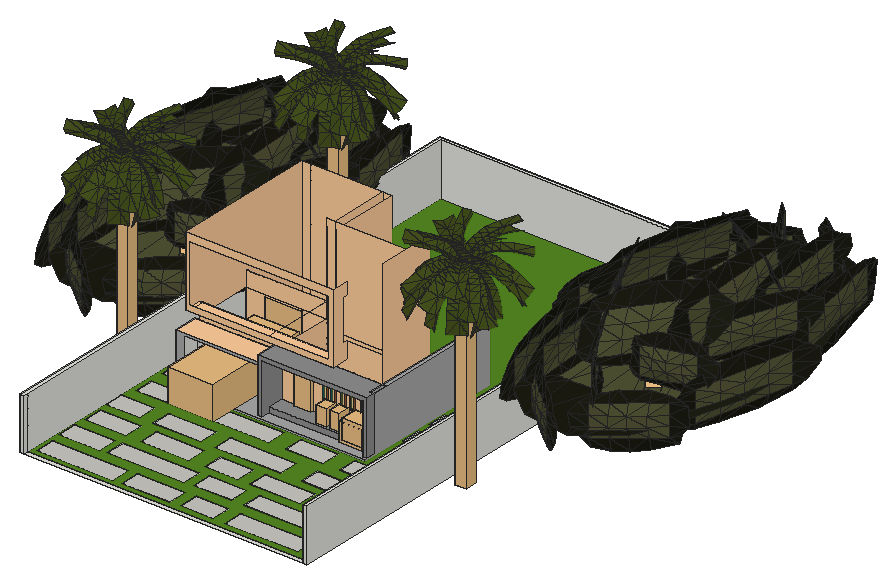
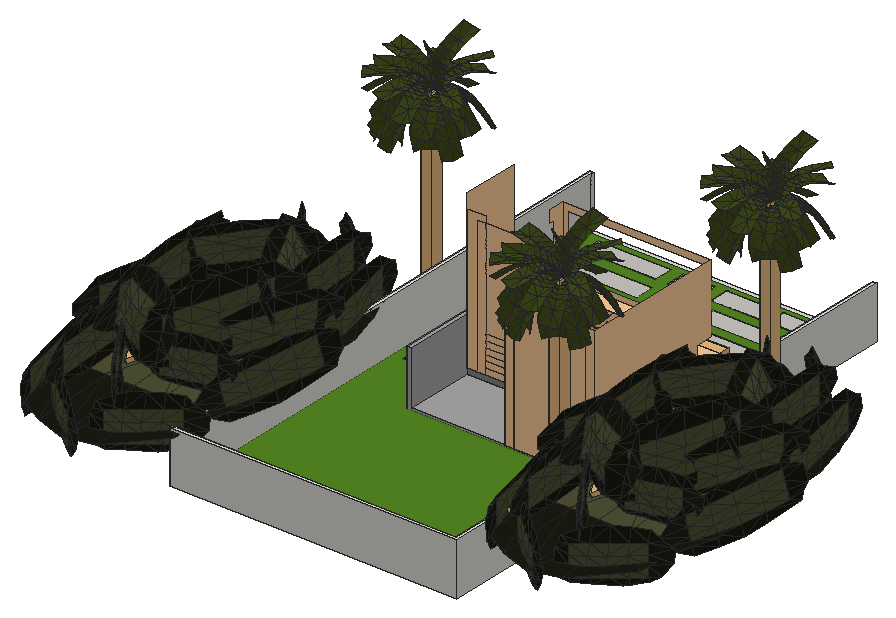
# SketchUp Ruby script. Lengths in inches.
U = 1.inch
M = Sketchup.active_model
def pt(a) = Geom::Point3d.new(a.map { |v| v * U })
def face(e, loops, mat)
  f = e.add_face(loops[0].map { |a| pt(a) })
  loops[1..].each { |l| e.add_face(l.map { |a| pt(a) }).erase! }
  f.material = f.back_material = mat if mat
  f
end
# faces: each face lists its corners as indices into pts; further lists are holes
def faces(e, pts, list, mat = nil) = list.each { |f| face(e, (f[0].is_a?(Array) ? f : [f]).map { |l| l.map { |i| pts[i] } }, mat) }
# xy, xz, yz: faces in a plane at the given z, y or x. An outline is a flat list of corners, or four numbers for a rectangle; further outlines are holes
def ring(l) = l.size == 4 ? [[l[0], l[1]], [l[2], l[1]], [l[2], l[3]], [l[0], l[3]]] : l.each_slice(2).to_a
def flat(e, list, mat, &to3) = list.each { |f| face(e, (f[0].is_a?(Array) ? f : [f]).map { |l| ring(l).map { |u, v| to3.(u, v) } }, mat) }
def xy(e, z, list, mat = nil) = flat(e, list, mat) { |x, y| [x, y, z] }
def xz(e, y, list, mat = nil) = flat(e, list, mat) { |x, z| [x, y, z] }
def yz(e, x, list, mat = nil) = flat(e, list, mat) { |y, z| [x, y, z] }
def lines(e, pts, list) = list.each { |a, b| e.add_line(pt(pts[a]), pt(pts[b])) }
# prism: a flat outline (further loops are holes) pulled along v
def prism(e, loops, v, mat = nil)
  f = face(e, loops, mat); d = Geom::Vector3d.new(v.map { |x| x * U })
  f.pushpull(f.normal.samedirection?(d) ? d.length : -d.length)
end
def box(e, o, s, mat = nil) = prism(e, [[o, [o[0] + s[0], o[1], o[2]], [o[0] + s[0], o[1] + s[1], o[2]], [o[0], o[1] + s[1], o[2]]]], [0, 0, s[2]], mat)
def at(x, y, z, deg = 0) = Geom::Transformation.translation(pt([x, y, z])) * Geom::Transformation.rotation(ORIGIN, Z_AXIS, deg.degrees)
def axes(o, x, y, z) = Geom::Transformation.new([*x, 0, *y, 0, *z, 0, *pt(o).to_a, 1])
def part(name) = M.definitions.add(name)
# library, detail: a bought-in or finely detailed component or shape, given as its bounding box
def library(name, o, s) = part(name).tap { |d| box(d.entities, o, s) }
def detail(e, o, s) = box(e.add_group.entities, o, s)
def put(e, d, t, mat = nil) = e.add_instance(d, t).tap { |i| i.material = mat if mat }
def group(e, t, mat = nil) = e.add_group.tap { |g| g.transformation = t; g.material = mat if mat }.entities
root = M.entities
M.materials.add("Brick_14_1K").color = [201, 199, 193]
M.materials.add("C02_Golden_Beige").color = [255, 205, 155]
M.materials.add("Glass_Basic_01").color = [176, 211, 103]
M.materials["Glass_Basic_01"].alpha = 0.25
M.materials.add("M03_Pewter_Shine").color = [168, 168, 168]
M.materials.add("M04_Stone_Frost").color = [142, 142, 142]
M.materials.add("Oak100_bottom").color = [27, 27, 17]
M.materials.add("Oak100_middle2").color = [80, 82, 52]
M.materials.add("Oak100_rs").color = [30, 31, 20]
M.materials.add("Oak100_top").color = [27, 27, 19]
M.materials.add("[0042_Sienna]").color = [160, 82, 45]
M.materials.add("[Color_004]").color = [176, 174, 161]
M.materials.add("[Color_F17]").color = [77, 130, 25]
M.materials["[Color_F17]"].alpha = 0.96
M.materials.add("[Color_H12]").color = [30, 153, 153]
M.materials.add("[Color_H17]").color = [20, 102, 102]
M.materials.add("[Color_H21]").color = [0, 51, 51]
M.materials.add("oak100_ls").color = [26, 27, 18]
M.materials.add("palmleaf").color = [66, 78, 27]
c1 = part("oak301branch")
detail(c1.entities,[0,-0.89,-1.57],[71.59,23.14,154.31])
c2 = part("center")
p = [[110.38,-8.75,48.08],[55.19,-7.5,48.08],[55.19,0,0.51],[110.38,0,0.51],[165.57,0,0.51],[165.57,-5.5,48.08],
  [0,0,48.08],[0,0,0.51],[220.76,0,0.51],[220.76,0,48.08],[110.38,-9,96.42],[55.19,-8,96.42],
  [165.57,-5,96.42],[0,0,96.42],[220.76,0,96.42],[110.38,0,144.75],[55.19,0,144.75],[165.57,0,144.75],
  [0,0,144.75],[220.76,0,144.75]]
faces(c2.entities,p,[[0,1,2],[0,2,3],[0,3,4],[0,4,5],[1,6,7],[1,7,2],[5,4,8],[5,8,9],
  [0,10,11],[0,12,10],[0,11,1],[0,5,12],[1,11,13],[1,13,6],[12,5,9],[12,9,14],
  [10,15,16],[10,16,11],[10,12,17],[10,17,15],[11,16,18],[11,18,13],[12,14,19],[12,19,17]],"Oak100_middle2")
c3 = part("leftside")
p = [[-0.5,8.25,24.35],[16,4.5,0],[47.5,0,0],[47.5,0,48.08],[-0.01,12.25,116.11],[47.5,0,96.42],
  [47.5,0,143.74],[16,6.25,143.74]]
faces(c3.entities,p,[[0,1,2],[0,2,3],[4,0,3],[4,3,5],[4,5,6],[4,6,7]],"oak100_ls")
c4 = part("rightside")
p = [[31.5,6,0],[63.6875,8.75,48.09],[0,0,48.08],[0,0,0],[62.93,15,107.53],[0,0,96.42],
  [0,0,144.75],[31.5,9.125,144.75]]
faces(c4.entities,p,[[0,1,2],[0,2,3],[1,4,5],[1,5,2],[4,6,5],[4,7,6]],"Oak100_rs")
c5 = part("top")
p = [[0,6.25,0],[31.5,0,0],[6.4,6,30.57],[86.69,0,0],[88.26,11.61,60.46],[141.83,8.25,66.91],
  [141.88,0,0],[197.07,0,0],[197.03,7.75,59.96],[252.26,0,0],[252.26,8.625,47.49],[283.76,9.125,0]]
faces(c5.entities,p,[[0,1,2],[2,1,3],[2,3,4],[5,4,3],[5,3,6],[5,6,7],[5,7,8],[8,7,9],
  [8,9,10],[9,11,10]],"Oak100_top")
c6 = part("Bottom")
p = [[86.66,14,16.04],[175.7,11.01,11.4],[141.88,0,55.29],[197.07,0,55.29],[197.04,9.67,16.05],[31.5,5.5,31.79],
  [86.69,0,55.29],[252.26,8,31.79],[252.26,0,55.29],[31.5,0,55.29],[0,4.5,55.29],[283.76,6,55.29]]
faces(c6.entities,p,[[0,1,2],[1,3,2],[1,4,3],[5,0,6],[0,2,6],[4,7,8],[4,8,3],[9,10,5],
  [5,6,9],[11,8,7]],"Oak100_bottom")
c7 = part("OakPatch_101b")
g1 = group(c7.entities,at(-25.67,-94.625,2.98))
put(g1,c2,axes([25.92,0,25.24],[0.54575,0,0],[0,0.5,0],[0,0,0.495]))
put(g1,c3,axes([0.75,0,25.24],[0.54575,0,0],[0,0.5,0],[0,0,0.495]))
put(g1,c4,axes([146.4,0,25.24],[0.54575,0,0],[0,0.5,0],[0,0,0.495]))
put(g1,c5,axes([8.73,0,96.4],[0.54575,0,0],[0,0.5,0],[0,0,0.495]))
put(g1,c6,axes([8.73,0,-1.875],[0.54575,0,0],[0,0.5,0],[0,0,0.495]))
c8 = part("big_oak_5")
put(c8.entities,c1,axes([-57.45,37.82,-17.01],[0.74533,-0.6144,0.25882],[0.63608,0.77162,0],[-0.19971,0.16463,0.96593]),"[Color_004]")
put(c8.entities,c1,axes([32.54,53.33,-17.01],[-0.60048,-0.7566,0.25882],[0.78329,-0.62166,0],[0.1609,0.20273,0.96593]),"[Color_004]")
put(c8.entities,c1,axes([41.42,-35.94,-18.75],[-0.70806,0.54087,0.45399],[0.67972,0.69627,0.23061],[0.19137,-0.47187,0.86065]),"[Color_004]")
put(c8.entities,c1,axes([-33.95,-51.625,-4.62],[0.48588,0.79631,0.3603],[-0.76814,0.58572,-0.25865],[-0.41699,-0.15109,0.89626]),"[Color_004]")
put(c8.entities,c7,at(-57.42,-78.66,64.97,-23.1))
put(c8.entities,c7,axes([135.88,-46.6,193.72],[-0.92784,-0.37299,0],[-0.37299,0.92784,0],[0,0,-1]))
put(c8.entities,c7,at(77.88,-55.71,54.47,66.9))
put(c8.entities,c7,axes([45.83,137.59,193.72],[0.37299,-0.92784,0],[-0.92784,-0.37299,0],[0,0,-1]))
put(c8.entities,c7,at(54.9375,79.58,54.47,156.9))
put(c8.entities,c7,at(-17.46,96.13,54.47,-158.1))
put(c8.entities,c7,axes([-127.27,-53.34,213.39],[0.38823,0.91019,-0.14436],[0.91982,-0.39234,0],[-0.05664,-0.13278,-0.98953]))
put(c8.entities,c7,at(-97.16,-15.76,73.97,-68.1))
put(c8.entities,c7,axes([15.22,-37.18,124.07],[0.72642,-0.53556,0],[0.53556,0.72642,0],[0,0,0.9025]))
put(c8.entities,c7,axes([37.03,-16.36,124.07],[0.89235,0.13496,0],[-0.13496,0.89235,0],[0,0,0.9025]))
put(c8.entities,c7,axes([37.72,13.79,124.07],[0.53556,0.72642,0],[-0.72642,0.53556,0],[0,0,0.9025]))
put(c8.entities,c7,axes([16.9,35.6,124.07],[-0.13496,0.89235,0],[-0.89235,-0.13496,0],[0,0,0.9025]))
put(c8.entities,c7,axes([-13.25,36.29,124.07],[-0.72642,0.53556,0],[-0.53556,-0.72642,0],[0,0,0.9025]))
put(c8.entities,c7,axes([-35.06,15.47,124.07],[-0.89235,-0.13496,0],[0.13496,-0.89235,0],[0,0,0.9025]))
put(c8.entities,c7,axes([-35.75,-14.68,124.07],[-0.53556,-0.72642,0],[0.72642,-0.53556,0],[0,0,0.9025]))
put(c8.entities,c7,axes([-14.93,-36.49,124.07],[0.13496,-0.89235,0],[0.89235,0.13496,0],[0,0,0.9025]))
put(c8.entities,c7,axes([-140.77,-218.68,-91.92],[2.2439,0,0],[0,0,-2.2439],[0,3.27968,0]))
put(c8.entities,c7,axes([-61.57,39.87,129.43],[0.8001,-0.8001,0],[0.77284,0.77284,-0.29286],[0.20708,0.20708,1.09296]))
put(c8.entities,c7,axes([-63.87,-48.04,129.43],[0.93696,0.63437,0],[-0.61275,0.90503,-0.29286],[-0.16419,0.2425,1.09296]))
put(c8.entities,c7,axes([6.15,-69.87,140.61],[-0.11631,1.12552,0],[-1.11537,-0.11526,-0.15161],[-0.1508,-0.01558,1.12131]))
put(c8.entities,c7,axes([67.89,-14.33,129.43],[-1.09556,0.28297,0],[-0.27333,-1.05823,-0.29286],[-0.07324,-0.28355,1.09296]))
put(c8.entities,c7,axes([17.19,57.86,129.43],[-0.56576,-0.97992,0],[0.94653,-0.54648,-0.29286],[0.25362,-0.14643,1.09296]))
c9 = part("palmleaf")
p = [[16.43,119.68,0],[0.28,119.68,7.08],[16.92,87.97,12.63],[36.77,119.68,4.95],[36.49,87.97,17.59],[18.25,0,6.49],
  [17.78,24.78,17.21],[0,0,13.57],[36.49,0,11.44],[0,87.97,19.71],[36.49,24.78,22.16],[0,64.81,26.16],
  [16.92,64.81,19.08],[36.49,64.81,24.03],[0,24.78,24.29],[17.52,38.05,19.67],[0,51.55,26.75],[17.52,51.55,19.67],
  [36.49,51.55,24.625],[0,38.05,26.75],[36.49,38.05,24.625]]
faces(c9.entities,p,[[0,1,2],[0,2,3],[4,3,2],[5,6,7],[5,8,6],[9,2,1],[10,6,8],[9,11,2],
  [12,2,11],[12,13,2],[4,2,13],[14,7,6],[6,15,14],[6,10,15],[11,16,12],[17,12,16],
  [17,18,12],[13,12,18],[19,14,15],[20,15,10],[16,19,17],[15,17,19],[15,20,17],[18,17,20]],"palmleaf")
c10 = part("palmleaf\#1")
p = [[16.43,119.68,0],[0.28,119.68,7.08],[16.92,87.97,12.63],[36.77,119.68,4.95],[36.49,87.97,17.59],[18.25,0,6.49],
  [17.78,24.78,17.21],[0,0,13.57],[36.49,0,11.44],[0,87.97,19.71],[36.49,24.78,22.16],[0,64.81,26.16],
  [16.92,64.81,19.08],[36.49,64.81,24.03],[0,24.78,24.29],[17.52,38.05,19.67],[0,51.55,26.75],[17.52,51.55,19.67],
  [36.49,51.55,24.625],[0,38.05,26.75],[36.49,38.05,24.625]]
faces(c10.entities,p,[[0,1,2],[0,2,3],[4,3,2],[5,6,7],[5,8,6],[9,2,1],[10,6,8],[9,11,2],
  [12,2,11],[12,13,2],[4,2,13],[14,7,6],[6,15,14],[6,10,15],[11,16,12],[17,12,16],
  [17,18,12],[13,12,18],[19,14,15],[20,15,10],[16,19,17],[15,17,19],[15,20,17],[18,17,20]],"palmleaf")
c11 = part("FF_tree_coconutpalm04")
g2 = group(c11.entities,at(20.16,13.1875,0))
detail(g2,[-29.3,-13.1875,0],[26.13,26.9375,457.72])
g3 = group(c11.entities,at(56.28,182.53,321.13))
put(g3,c9,axes([-71.46,-195.01,116.18],[0.73937,0.73944,-0.22966],[-0.71356,0.52745,-0.59901],[-0.30058,0.56675,0.8571]))
put(g3,c9,axes([-68.01,-171.32,127.68],[1.04922,-0.18505,0.10525],[0.15991,1.03447,0.22468],[-0.14053,-0.20447,1.04145]))
put(g3,c9,axes([-64.72,-189.21,117.32],[0.64626,0.81802,0.24368],[-0.84975,0.58782,0.28032],[0.08039,-0.36262,1.0041]))
put(g3,c9,axes([-43.1875,-192.71,115.26],[-0.56113,0.86864,0.2771],[-0.65162,-0.60964,0.59154],[0.63774,0.14138,0.84823]))
put(g3,c9,axes([-67.54,-179.99,121.34],[1.04522,0.23172,0],[-0.23172,1.04522,0],[0,0,1.0706]))
put(g3,c9,axes([-38.56,-158.65,128.63],[-0.37037,-0.97449,0.24368],[0.98718,-0.30509,0.28032],[-0.18571,0.32167,1.0041]))
put(g3,c9,axes([-60.15,-161.79,126.57],[0.79636,-0.6597,0.2771],[0.43814,0.77737,0.59154],[-0.56571,-0.32661,0.84823]))
put(g3,c9,axes([-33.09,-166.59,132.64],[-0.92717,-0.5353,0],[0.5353,-0.92717,0],[0,0,1.0706]))
put(g3,c10,axes([-36.87,-167.81,105.66],[-0.92717,-0.5353,0],[0.22453,-0.3889,-0.7289],[0.48593,-0.84166,0.3368]))
put(g3,c9,axes([-66.8,-168.47,116.57],[1.04948,-0.21161,0],[0.169,0.83815,-0.6443],[0.12735,0.63159,0.85502]))
put(g3,c9,axes([-47.72,-145.76,141],[0.06161,-1.03598,-0.26295],[1.00548,0.1455,-0.33768],[0.3625,-0.22752,0.98133]))
put(g3,c9,axes([-43.65,-167.17,115.4375],[-0.10718,-0.78652,0.71839],[0.91876,-0.43363,-0.33768],[0.53905,0.58269,0.71839]))
put(g3,c9,axes([-27.17,-189.68,131.6],[-1.05022,0.18096,-0.10237],[-0.19666,-0.69362,0.79145],[0.06745,0.79519,0.71366]))
put(g3,c10,axes([-38.11,-198.32,130.88],[-0.11191,1.06474,0],[-0.53845,-0.05659,-0.7761],[-0.89174,-0.09373,0.30245]))
put(g3,c10,axes([-58.14,-186.45,115.23],[0.77414,0.73902,0.02061],[-0.13343,0.1787,-0.78534],[-0.72739,0.75373,0.16599]))
put(g3,c10,axes([-64.06,-165.8,117.18],[0.92056,-0.54659,0],[0.24303,0.40931,-0.71921],[0.48958,0.82455,0.35702]))
put(g3,c10,axes([-57.75,-156.01,93.65],[0.12988,-1.06234,0.02061],[0.22302,0.00018,-0.78534],[1.03903,0.13276,0.16599]))
put(g3,c9,axes([-58.5,-171.33,127.28],[0.97557,-0.23867,0.37079],[0.42622,0.74121,-0.6443],[-0.11307,0.73473,0.77044]))
put(g3,c9,axes([-44.51,-184.55,127.28],[-0.77889,0.63406,0.37079],[-0.70295,-0.48674,-0.6443],[-0.21301,-0.71221,0.77044]))
put(g3,c9,axes([-36.71,-172.91,109.98],[-1.02609,-0.14726,0.26765],[0.06816,-0.92821,-0.24938],[0.29595,-0.24664,0.99888]))
put(g3,c9,axes([-41.84,-171.13,127.28],[-0.6143,-0.71527,0.37079],[0.42829,-0.40094,-0.6443],[0.65381,0.00894,0.77044]))
put(g3,c9,axes([-59.17,-160.07,127.68],[0.61106,-0.87276,0.10525],[0.84455,0.61841,0.22468],[-0.24395,-0.04521,1.04145]))
put(g3,c9,axes([-55.27,-168.02,127.28],[0.75974,-0.65688,0.37079],[0.71708,0.46568,-0.6443],[0.23404,0.70557,0.77044]))
put(g3,c9,axes([-61.37,-161.6875,116.57],[0.83786,-0.66646,0],[0.53226,0.66914,-0.6443],[0.40109,0.50424,0.85502]))
put(g3,c9,axes([-35.93,-165.13,116.57],[-0.62365,-0.77418,0],[0.61827,-0.21591,-0.6443],[0.4659,-0.1627,0.85502]))
put(g3,c9,axes([-32.62,-180.6,121.34],[-1.04358,0.23901,0],[-0.23901,-1.04358,0],[0,0,1.0706]))
put(g3,c9,axes([-60.55,-185.18,109.98],[0.86374,0.57315,0.26765],[-0.45972,0.80925,-0.24938],[-0.37313,0.09585,0.99888]))
put(g3,c9,axes([-38.23,-190.69,116.57],[-0.85726,0.64131,0],[-0.51218,-0.68464,-0.6443],[-0.38595,-0.51591,0.85502]))
put(g3,c9,axes([-53.45,-197.7,123],[0.22225,1.04446,-0.07672],[-0.86366,0.15654,-0.37078],[-0.39383,0.15603,0.98323]))
put(g3,c10,axes([-36.75,-178.79,102.19],[-1.00197,0.37183,-0.04734],[-0.14939,-0.55582,-0.67705],[-0.3463,-0.83605,0.42906]))
put(g3,c9,axes([-63.02,-150.39,128.6],[0.94003,-0.47987,0.17959],[-0.10261,0.1027,0.81148],[-0.49474,-0.94769,0.05738]))
c12 = library("BMW",[-132.24,-54.45,0],[229.73,90.4,71.64])
c13 = library("Plant Banana",[-25.32,5.73,12.47],[52.12,39.56,44.04])
c14 = library("porta de madeira",[3.7,-4.82,1.36],[53.55,7.65,83.26])
c15 = library("Amelie+Madeira",[-106.62,-9.14,57.07],[22.04,26.92,33.38])
c16 = part("okno 2094 st 1")
xy(c16.entities,0,[[55.59,77.87,83.07,85.74]],"[0042_Sienna]")
xy(c16.entities,1.18,[[56.77,79.84,81.89,83.77]])
xy(c16.entities,1.18,[[56.77,77.87,81.89,79.84],[56.77,83.77,81.89,85.74]],"[Color_H21]")
xy(c16.entities,1.57,[[57.16,79.84,81.49,81.8],[57.16,81.8,81.49,83.77]],"[Color_H21]")
xy(c16.entities,80.87,[[57.16,79.84,81.49,81.8],[57.16,81.8,81.49,83.77]],"[Color_H17]")
xy(c16.entities,81.26,[[56.77,79.84,81.89,83.77]])
xy(c16.entities,81.26,[[56.77,77.87,81.89,79.84],[56.77,83.77,81.89,85.74]],"[Color_H17]")
xy(c16.entities,82.44,[[55.59,77.87,83.07,85.74]],"[0042_Sienna]")
xz(c16.entities,77.87,[[[55.59,0,83.07,82.44],[56.77,1.18,81.89,81.26]]],"[Color_H17]")
xz(c16.entities,79.84,[[[56.77,1.18,81.89,81.26],[57.16,1.57,81.49,80.87]]],"[Color_H12]")
xz(c16.entities,81.8,[[57.16,1.57,81.49,80.87]],"Glass_Basic_01")
xz(c16.entities,83.77,[[[56.77,1.18,81.89,81.26],[57.16,1.57,81.49,80.87]]],"[Color_H12]")
xz(c16.entities,85.74,[[[55.59,0,83.07,82.44],[56.77,1.18,81.89,81.26]]],"[Color_H17]")
yz(c16.entities,55.59,[[77.87,0,85.74,82.44]],"[0042_Sienna]")
yz(c16.entities,56.77,[[79.84,1.18,83.77,81.26]])
yz(c16.entities,56.77,[[77.87,1.18,79.84,81.26],[83.77,1.18,85.74,81.26]],"[Color_H17]")
yz(c16.entities,57.16,[[79.84,1.57,81.8,80.87],[81.8,1.57,83.77,80.87]],"[Color_H17]")
yz(c16.entities,81.49,[[79.84,1.57,81.8,80.87],[81.8,1.57,83.77,80.87]],"[Color_H17]")
yz(c16.entities,81.89,[[79.84,1.18,83.77,81.26]])
yz(c16.entities,81.89,[[77.87,1.18,79.84,81.26],[83.77,1.18,85.74,81.26]],"[Color_H17]")
yz(c16.entities,83.07,[[77.87,0,85.74,82.44]],"[0042_Sienna]")
c17 = library("Windows_Triple-Wood-Casement-Window-51inx36in",[0,0,-2.19],[51,41,3.19])
xy(root,0,[[381.1875,0,1020.73,9]])
xy(root,0,[[[381.1875,9,1020.73,1194.87],[807.59,98.08,1014.79,143.57],[392.14,22.02,567.51,67.52],[523.44,304.32,698.8125,349.82],[832.74,231.78,1008.11,277.28],[496.28,94.38,671.65,139.88],[822.76,24.99,988.82,70.48],[635.27,230.42,785.07,275.92],[767.04,164.08,881.8125,209.58],[882.6,458.86,994.98,504.36],[882.6,535.24,994.98,580.73],[861.27,304.32,972.36,349.82],[517.56,164.08,628.64,209.58],[888.67,382.19,999.76,427.6875],[492.77,230.69,601.38,276.1875],[587.35,23.23,695.96,68.73],[900.9375,164.08,1003.41,209.58],[388.79,163.875,482.48,209.37],[386.4,92.65,480.09,138.15],[737.2,304.32,822.9,349.82],[692.58,98.08,778.27,143.57],[394.4,304.32,480.09,349.82],[383.27,230.69,460.96,276.1875],[719.85,24.99,794.7,70.48],[665.36,164.08,740.2,209.58],[392.29,381.15,433.52,426.64],[392.29,458.125,433.52,503.625]]],"[Color_F17]")
xy(root,0.97,[[392.14,22.02,567.51,67.52],[587.35,23.23,695.96,68.73],[719.85,24.99,794.7,70.48],[822.76,24.99,988.82,70.48],[386.4,92.65,480.09,138.15],
  [496.28,94.38,671.65,139.88],[692.58,98.08,778.27,143.57],[807.59,98.08,1014.79,143.57],[388.79,163.875,482.48,209.37],[517.56,164.08,628.64,209.58],
  [665.36,164.08,740.2,209.58],[767.04,164.08,881.8125,209.58],[900.9375,164.08,1003.41,209.58],[635.27,230.42,785.07,275.92],[383.27,230.69,460.96,276.1875],
  [492.77,230.69,601.38,276.1875],[832.74,231.78,1008.11,277.28],[394.4,304.32,480.09,349.82],[523.44,304.32,698.8125,349.82],[737.2,304.32,822.9,349.82],
  [861.27,304.32,972.36,349.82],[392.29,381.15,433.52,426.64],[888.67,382.19,999.76,427.6875],[392.29,458.125,433.52,503.625],[882.6,458.86,994.98,504.36],
  [882.6,535.24,994.98,580.73]],"Brick_14_1K")
xy(root,4,[[435.93,365.38,456.73,400.96]])
xy(root,4,[[445.59,556.1875,630.52,716.63]],"C02_Golden_Beige")
xy(root,16.58,[[630.52,422.1,630.52,556.1875,866.19,556.1875,866.19,422.1,705.91,422.1,705.91,425.36,667,425.36,667,422.1]],"C02_Golden_Beige")
xy(root,40.04,[[488.67,556.1875,573.91,560.17]],"C02_Golden_Beige")
xy(root,108.26,[[667,422.1,705.91,425.36]],"C02_Golden_Beige")
xy(root,113.14,[[435.93,365.38,624.21,422.1]],"C02_Golden_Beige")
xy(root,116.43,[[488.67,556.1875,573.91,560.17]],"C02_Golden_Beige")
xy(root,120,[[372.1875,0,381.1875,0,381.1875,1194.87,1020.73,1194.87,1020.73,0,1029.73,0,1029.73,1203.87,372.1875,1203.87]])
xy(root,151.45,[[445.59,382.49,453.59,422.1],[453.59,382.49,622.52,422.1],[622.52,382.49,784.98,422.1]],"C02_Golden_Beige")
xy(root,157.52,[[445.59,555.98,630.52,556.1875]],"C02_Golden_Beige")
xz(root,0,[[372.1875,0,381.1875,120],[1020.73,0,1029.73,120]])
xz(root,22.02,[[392.14,0,567.51,0.97]])
xz(root,23.23,[[587.35,0,695.96,0.97]])
xz(root,24.99,[[719.85,0,794.7,0.97],[822.76,0,988.82,0.97]])
xz(root,67.52,[[392.14,0,567.51,0.97]])
xz(root,68.73,[[587.35,0,695.96,0.97]])
xz(root,70.48,[[719.85,0,794.7,0.97],[822.76,0,988.82,0.97]])
xz(root,92.65,[[386.4,0,480.09,0.97]])
xz(root,94.38,[[496.28,0,671.65,0.97]])
xz(root,98.08,[[692.58,0,778.27,0.97],[807.59,0,1014.79,0.97]])
xz(root,138.15,[[386.4,0,480.09,0.97]])
xz(root,139.88,[[496.28,0,671.65,0.97]])
xz(root,143.57,[[692.58,0,778.27,0.97],[807.59,0,1014.79,0.97]])
xz(root,163.875,[[388.79,0,482.48,0.97]])
xz(root,164.08,[[517.56,0,628.64,0.97],[665.36,0,740.2,0.97],[767.04,0,881.8125,0.97],[900.9375,0,1003.41,0.97]])
xz(root,209.37,[[388.79,0,482.48,0.97]])
xz(root,209.58,[[517.56,0,628.64,0.97],[665.36,0,740.2,0.97],[767.04,0,881.8125,0.97],[900.9375,0,1003.41,0.97]])
xz(root,230.42,[[635.27,0,785.07,0.97]])
xz(root,230.69,[[383.27,0,460.96,0.97],[492.77,0,601.38,0.97]])
xz(root,231.78,[[832.74,0,1008.11,0.97]])
xz(root,275.92,[[635.27,0,785.07,0.97]])
xz(root,276.1875,[[383.27,0,460.96,0.97],[492.77,0,601.38,0.97]])
xz(root,277.28,[[832.74,0,1008.11,0.97]])
xz(root,304.32,[[394.4,0,480.09,0.97],[523.44,0,698.8125,0.97],[737.2,0,822.9,0.97],[861.27,0,972.36,0.97]])
xz(root,349.82,[[394.4,0,480.09,0.97],[523.44,0,698.8125,0.97],[737.2,0,822.9,0.97],[861.27,0,972.36,0.97]])
xz(root,365.38,[[435.93,4,456.73,4,456.73,107.87,624.21,107.87,624.21,113.14,435.93,113.14]],"M03_Pewter_Shine")
xz(root,381.15,[[392.29,0,433.52,0.97]])
xz(root,382.19,[[888.67,0,999.76,0.97]])
xz(root,382.49,[[[445.59,151.45,784.98,311.04],[453.59,164.34,774.4375,295.51]]],"C02_Golden_Beige")
xz(root,400.96,[[435.93,4,456.73,107.88]])
xz(root,422.1,[[630.52,16.58,667,16.58,667,108.26,705.91,108.26,705.91,16.58,866.19,16.58,866.19,189.3,784.98,189.3,784.98,151.45,445.59,151.45,445.59,113.14,624.21,113.14,624.21,121.39,630.52,121.39],[435.93,107.87,624.21,113.14]],"C02_Golden_Beige")
xz(root,425.36,[[667,16.58,705.91,108.26]],"C02_Golden_Beige")
xz(root,426.64,[[392.29,0,433.52,0.97]])
xz(root,427.6875,[[888.67,0,999.76,0.97]])
xz(root,458.125,[[392.29,0,433.52,0.97]])
xz(root,458.86,[[882.6,0,994.98,0.97]])
xz(root,503.625,[[392.29,0,433.52,0.97]])
xz(root,504.36,[[882.6,0,994.98,0.97]])
xz(root,535.24,[[882.6,0,994.98,0.97]])
xz(root,555.98,[[445.59,121.39,630.52,157.52]],"C02_Golden_Beige")
xz(root,556.1875,[[651.625,2.29,651.625,2.33,845.09,2.33,845.09,16.58,866.19,16.58,866.19,2.29],[630.52,2.33,651.625,16.58],[651.625,2.33,845.09,16.58],[[445.59,4,630.52,157.52],[488.67,40.04,573.91,116.43]],[630.52,16.58,651.625,30.72],
  [651.625,16.58,823.98,30.72],[823.98,16.58,845.09,328.72],[845.09,16.58,845.09,328.72,823.98,328.72,823.98,342.97,866.19,342.97,866.19,16.58],[630.52,30.72,651.625,44.85],[651.625,30.72,823.98,44.85],
  [630.52,44.85,651.625,58.98],[651.625,44.85,823.98,58.98],[630.52,58.98,651.625,73.12],[651.625,58.98,823.98,73.12],[630.52,73.12,651.625,87.25],
  [651.625,73.12,823.98,87.25],[630.52,87.25,651.625,101.38],[651.625,87.25,823.98,101.38],[630.52,101.38,651.625,328.72],[651.625,101.38,823.98,328.72]],"C02_Golden_Beige")
xz(root,560.17,[[488.67,40.04,573.91,116.43]],"C02_Golden_Beige")
xz(root,580.73,[[882.6,0,994.98,0.97]])
xz(root,716.63,[[445.59,4,466.69,311.04],[466.69,4,630.52,311.04],[630.52,4,651.625,311.04]],"C02_Golden_Beige")
xz(root,1194.87,[[381.1875,0,1020.73,120]])
xz(root,1203.87,[[372.1875,0,1029.73,120]])
yz(root,372.1875,[[0,0,1203.87,120]])
yz(root,381.1875,[[0,0,9,120],[9,0,1194.87,120]])
yz(root,383.27,[[230.69,0,276.1875,0.97]])
yz(root,386.4,[[92.65,0,138.15,0.97]])
yz(root,388.79,[[163.875,0,209.37,0.97]])
yz(root,392.14,[[22.02,0,67.52,0.97]])
yz(root,392.29,[[381.15,0,426.64,0.97],[458.125,0,503.625,0.97]])
yz(root,394.4,[[304.32,0,349.82,0.97]])
yz(root,433.52,[[381.15,0,426.64,0.97],[458.125,0,503.625,0.97]])
yz(root,435.93,[[365.38,107.87,400.96,107.88]])
yz(root,435.93,[[365.38,4,400.96,107.87],[400.96,107.87,400.96,107.88,365.38,107.88,365.38,113.14,422.1,113.14,422.1,107.87]],"M03_Pewter_Shine")
yz(root,445.59,[[556.1875,4,556.1875,157.52,555.98,157.52,555.98,121.39,422.1,121.39,422.1,151.45,382.49,151.45,382.49,311.04,716.63,311.04,716.63,4]],"C02_Golden_Beige")
yz(root,456.73,[[365.38,4,400.96,107.88]])
yz(root,460.96,[[230.69,0,276.1875,0.97]])
yz(root,480.09,[[92.65,0,138.15,0.97],[304.32,0,349.82,0.97]])
yz(root,482.48,[[163.875,0,209.37,0.97]])
yz(root,488.67,[[556.1875,40.04,560.17,116.43]],"C02_Golden_Beige")
yz(root,492.77,[[230.69,0,276.1875,0.97]])
yz(root,496.28,[[94.38,0,139.88,0.97]])
yz(root,517.56,[[164.08,0,209.58,0.97]])
yz(root,523.44,[[304.32,0,349.82,0.97]])
yz(root,567.51,[[22.02,0,67.52,0.97]])
yz(root,573.91,[[556.1875,40.04,560.17,116.43]],"C02_Golden_Beige")
yz(root,587.35,[[23.23,0,68.73,0.97]])
yz(root,601.38,[[230.69,0,276.1875,0.97]])
yz(root,624.21,[[365.38,107.87,422.1,113.14]],"C02_Golden_Beige")
yz(root,628.64,[[164.08,0,209.58,0.97]])
yz(root,630.52,[[556.1875,4,716.63,311.04],[422.1,16.58,422.1,121.39,555.98,121.39,555.98,157.52,556.1875,157.52,556.1875,16.58]],"C02_Golden_Beige")
yz(root,635.27,[[230.42,0,275.92,0.97]])
yz(root,651.625,[[556.1875,4,716.63,311.04]],"C02_Golden_Beige")
yz(root,665.36,[[164.08,0,209.58,0.97]])
yz(root,667,[[422.1,16.58,425.36,108.26]],"C02_Golden_Beige")
yz(root,671.65,[[94.38,0,139.88,0.97]])
yz(root,692.58,[[98.08,0,143.57,0.97]])
yz(root,695.96,[[23.23,0,68.73,0.97]])
yz(root,698.8125,[[304.32,0,349.82,0.97]])
yz(root,705.91,[[422.1,16.58,425.36,108.26]],"C02_Golden_Beige")
yz(root,719.85,[[24.99,0,70.48,0.97]])
yz(root,737.2,[[304.32,0,349.82,0.97]])
yz(root,740.2,[[164.08,0,209.58,0.97]])
yz(root,767.04,[[164.08,0,209.58,0.97]])
yz(root,778.27,[[98.08,0,143.57,0.97]])
yz(root,784.98,[[382.49,151.45,422.1,151.45,422.1,189.3,409.65,189.3,409.65,283.57,422.1,283.57,422.1,311.04,382.49,311.04]],"C02_Golden_Beige")
yz(root,785.07,[[230.42,0,275.92,0.97]])
yz(root,794.7,[[24.99,0,70.48,0.97]])
yz(root,807.59,[[98.08,0,143.57,0.97]])
yz(root,822.76,[[24.99,0,70.48,0.97]])
yz(root,822.9,[[304.32,0,349.82,0.97]])
yz(root,832.74,[[231.78,0,277.28,0.97]])
yz(root,861.27,[[304.32,0,349.82,0.97]])
yz(root,866.19,[[422.1,16.58,556.1875,376.07]],"C02_Golden_Beige")
yz(root,881.8125,[[164.08,0,209.58,0.97]])
yz(root,882.6,[[458.86,0,504.36,0.97],[535.24,0,580.73,0.97]])
yz(root,888.67,[[382.19,0,427.6875,0.97]])
yz(root,900.9375,[[164.08,0,209.58,0.97]])
yz(root,972.36,[[304.32,0,349.82,0.97]])
yz(root,988.82,[[24.99,0,70.48,0.97]])
yz(root,994.98,[[458.86,0,504.36,0.97],[535.24,0,580.73,0.97]])
yz(root,999.76,[[382.19,0,427.6875,0.97]])
yz(root,1003.41,[[164.08,0,209.58,0.97]])
yz(root,1008.11,[[231.78,0,277.28,0.97]])
yz(root,1014.79,[[98.08,0,143.57,0.97]])
yz(root,1020.73,[[0,0,9,120],[9,0,1194.87,120]])
yz(root,1029.73,[[0,0,1203.87,120]])
p = [[630.52,555.98,157.52],[630.52,422.1,157.52]]
lines(root,p,[[0,1]])
put(root,c8,axes([1180.59,905.7,0],[1,0,0],[0,2,0],[0,0,1]))
put(root,c8,axes([223.64,766.96,0],[1,0,0],[0,2,0],[0,0,1]))
put(root,c11,at(455.03,788.12,0))
put(root,c11,at(336.63,331.5,0))
put(root,c11,at(1063.61,395.22,0))
g4 = group(root,at(624.21,365.38,0),"M03_Pewter_Shine")
xy(g4,0,[[-188.28,-7.67,252.22,351.25]])
xy(g4,4,[[-188.28,-7.67,252.22,-7.67,252.22,20.47,241.98,20.47,241.98,351.25,-188.28,351.25]])
xy(g4,127.84,[[241.98,20.47,252.22,351.25]])
xz(g4,-7.67,[[-188.28,0,252.22,4]])
xz(g4,20.47,[[241.98,4,252.22,127.84]])
xz(g4,351.25,[[-188.28,0,-188.28,4,241.98,4,241.98,127.84,252.22,127.84,252.22,0]])
yz(g4,-188.28,[[-7.67,0,351.25,4]])
yz(g4,241.98,[[20.47,4,351.25,127.84]])
yz(g4,252.22,[[-7.67,0,351.25,0,351.25,127.84,20.47,127.84,20.47,4,-7.67,4]])
g5 = group(root,at(624.21,365.38,4),"M03_Pewter_Shine")
xy(g5,0,[[0,0,0,56.72,6.31,56.72,6.31,20.47,10.3,20.47,10.3,0],[241.52,0,251.82,20.47],[6.31,20.47,241.98,190.8125]],"M04_Stone_Frost")
xy(g5,12.58,[[10.3,20.47,241.98,20.47,241.98,190.8125,6.31,190.8125,6.31,56.72,10.3,56.72],[6.31,20.47,10.3,56.72]],"M04_Stone_Frost")
xy(g5,114.89,[[10.3,0,241.52,56.72]],"M04_Stone_Frost")
xy(g5,120,[[241.52,20.47,241.98,56.72],[241.98,20.47,247.83,56.72],[247.83,20.47,251.82,56.72]],"M04_Stone_Frost")
xy(g5,123.84,[[0,0,251.82,56.72]],"M04_Stone_Frost")
xz(g5,0,[[0,0,10.3,0,10.3,114.89,241.52,114.89,241.52,0,251.82,0,251.82,123.84,0,123.84]],"M04_Stone_Frost")
xz(g5,20.47,[[6.31,0,10.3,12.58],[10.3,0,241.52,12.58],[241.52,0,241.98,12.58],[241.98,0,247.83,120],[247.83,0,251.82,120],
  [241.52,12.58,241.98,120]],"M04_Stone_Frost")
xz(g5,56.72,[[0,0,0,123.84,10.3,123.84,10.3,12.58,6.31,12.58,6.31,0],[10.3,114.89,10.3,123.84,251.82,123.84,251.82,120,241.52,120,241.52,114.89]],"M04_Stone_Frost")
xz(g5,190.8125,[[6.31,0,241.98,12.58]],"M04_Stone_Frost")
yz(g5,0,[[0,0,56.72,123.84]],"M04_Stone_Frost")
yz(g5,6.31,[[20.47,0,56.72,12.58],[56.72,0,190.8125,12.58]],"M04_Stone_Frost")
yz(g5,10.3,[[0,0,20.47,0,20.47,12.58,56.72,12.58,56.72,114.89,0,114.89]],"M04_Stone_Frost")
yz(g5,241.52,[[0,0,20.47,114.89],[20.47,114.89,56.72,120]],"M04_Stone_Frost")
yz(g5,241.98,[[20.47,0,190.8125,12.58]],"M04_Stone_Frost")
yz(g5,251.82,[[0,0,20.47,0,20.47,120,56.72,120,56.72,123.84,0,123.84]],"M04_Stone_Frost")
put(root,c12,axes([536.1,401.32,4],[0,-1.07,0],[1.14,0,0],[0,0,1.07144]))
put(root,c13,at(824.23,374.68,-8.31))
put(root,c13,at(831.03,374.53,-0.98))
put(root,c14,axes([664.31,422.1,15.08],[0.72669,0,0],[0,1,0],[0,0,1.10116]))
put(root,c15,axes([857.69,401.36,-47.34],[1.13,0,0],[0,1,0],[0,0,1.12]))
put(root,c15,axes([875.04,401.36,-47.34],[1,0,0],[0,1,0],[0,0,1.12]))
put(root,c16,axes([799.625,396.2,26.16],[0.34565,0,0],[0,0.3021,0],[0,0,1.0224]))
put(root,c17,axes([488.67,556.1875,40.04],[1.67137,0,0],[0,0,1.86328],[0,-1,0]))
put(root,c16,axes([711.67,396.2,51.09],[0.34565,0,0],[0,0.3021,0],[0,0,0.72]))
put(root,c16,axes([729.72,396.2,51.09],[0.34565,0,0],[0,0.3021,0],[0,0,0.72]))
put(root,c16,axes([774.3125,396.2,51.09],[0.34565,0,0],[0,0.3021,0],[0,0,0.72]))
put(root,c16,axes([752.47,396.2,51.09],[0.34565,0,0],[0,0.3021,0],[0,0,0.72]))
